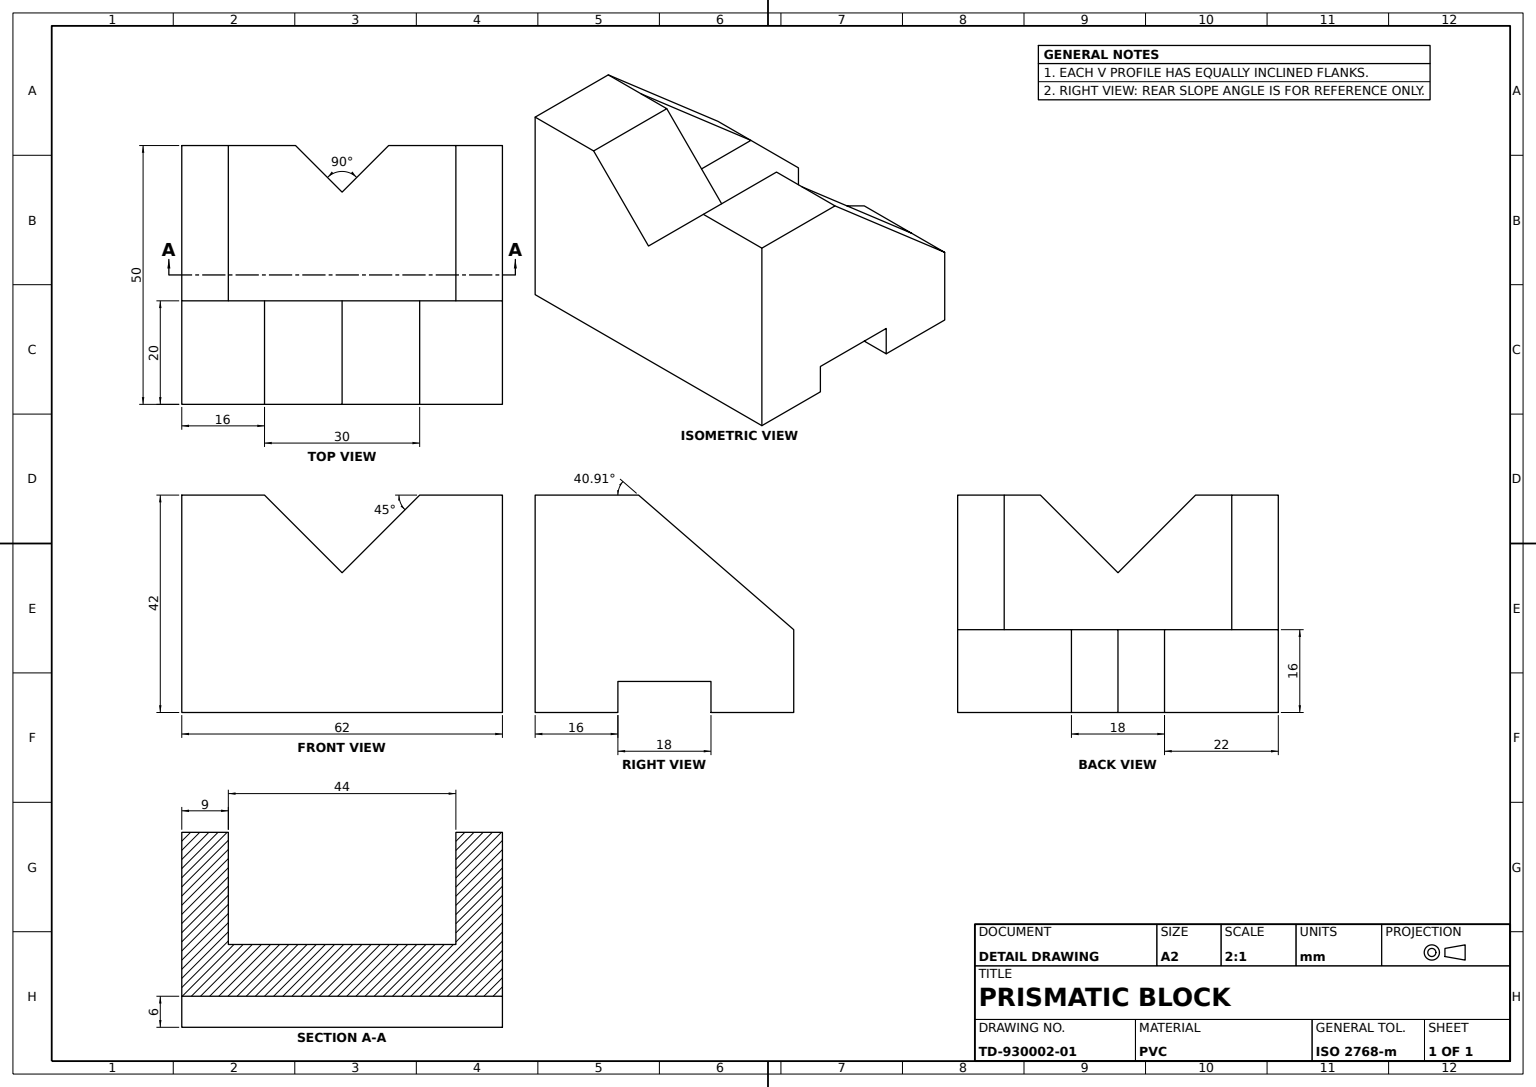
ISO-10303-21;
HEADER;
FILE_DESCRIPTION((''),'2;1');
FILE_NAME('','',(''),(''),'','','');
FILE_SCHEMA(('AUTOMOTIVE_DESIGN'));
ENDSEC;
DATA;
#1=APPLICATION_CONTEXT('');
#2=PRODUCT_CONTEXT('',#1,'mechanical');
#3=PRODUCT('','','',(#2));
#4=PRODUCT_DEFINITION_FORMATION('','',#3);
#5=PRODUCT_DEFINITION_CONTEXT('',#1,'design');
#6=PRODUCT_DEFINITION('','',#4,#5);
#7=PRODUCT_DEFINITION_SHAPE('','',#6);
#8=(LENGTH_UNIT()NAMED_UNIT(*)SI_UNIT(.MILLI.,.METRE.));
#9=(NAMED_UNIT(*)PLANE_ANGLE_UNIT()SI_UNIT($,.RADIAN.));
#10=(NAMED_UNIT(*)SI_UNIT($,.STERADIAN.)SOLID_ANGLE_UNIT());
#11=UNCERTAINTY_MEASURE_WITH_UNIT(LENGTH_MEASURE(0.005),#8,'distance_accuracy_value','');
#12=(GEOMETRIC_REPRESENTATION_CONTEXT(3)GLOBAL_UNCERTAINTY_ASSIGNED_CONTEXT((#11))GLOBAL_UNIT_ASSIGNED_CONTEXT((#8,#9,#10))REPRESENTATION_CONTEXT('',''));
#13=CARTESIAN_POINT('',(9.,25.,-21.));
#14=VERTEX_POINT('',#13);
#15=CARTESIAN_POINT('',(31.,25.,-21.));
#16=VERTEX_POINT('',#15);
#17=CARTESIAN_POINT('',(0.,25.,-21.));
#18=DIRECTION('',(1.,0.,0.));
#19=VECTOR('',#18,1000.);
#20=LINE('',#17,#19);
#21=EDGE_CURVE('',#14,#16,#20,.T.);
#22=ORIENTED_EDGE('',*,*,#21,.T.);
#23=CARTESIAN_POINT('',(31.,9.,-21.));
#24=VERTEX_POINT('',#23);
#25=CARTESIAN_POINT('',(31.,0.,-21.));
#26=DIRECTION('',(0.,1.,0.));
#27=VECTOR('',#26,1000.);
#28=LINE('',#25,#27);
#29=EDGE_CURVE('',#24,#16,#28,.T.);
#30=ORIENTED_EDGE('',*,*,#29,.F.);
#31=CARTESIAN_POINT('',(-31.,9.,-21.));
#32=VERTEX_POINT('',#31);
#33=CARTESIAN_POINT('',(0.,9.,-21.));
#34=DIRECTION('',(-1.,0.,0.));
#35=VECTOR('',#34,1000.);
#36=LINE('',#33,#35);
#37=EDGE_CURVE('',#24,#32,#36,.T.);
#38=ORIENTED_EDGE('',*,*,#37,.T.);
#39=CARTESIAN_POINT('',(-31.,25.,-21.));
#40=VERTEX_POINT('',#39);
#41=CARTESIAN_POINT('',(-31.,0.,-21.));
#42=LINE('',#41,#27);
#43=EDGE_CURVE('',#32,#40,#42,.T.);
#44=ORIENTED_EDGE('',*,*,#43,.T.);
#45=CARTESIAN_POINT('',(-9.,25.,-21.));
#46=VERTEX_POINT('',#45);
#47=EDGE_CURVE('',#40,#46,#20,.T.);
#48=ORIENTED_EDGE('',*,*,#47,.T.);
#49=CARTESIAN_POINT('',(0.,16.,-21.));
#50=VERTEX_POINT('',#49);
#51=DIRECTION('',(0.707106781,-0.707106781,0.));
#52=VECTOR('',#51,1000.);
#53=LINE('',#49,#52);
#54=EDGE_CURVE('',#46,#50,#53,.T.);
#55=ORIENTED_EDGE('',*,*,#54,.T.);
#56=CARTESIAN_POINT('',(-20.5,-4.5,-21.));
#57=DIRECTION('',(-0.707106781,-0.707106781,0.));
#58=VECTOR('',#57,1000.);
#59=LINE('',#56,#58);
#60=EDGE_CURVE('',#14,#50,#59,.T.);
#61=ORIENTED_EDGE('',*,*,#60,.F.);
#62=EDGE_LOOP('',(#22,#30,#38,#44,#48,#55,#61));
#63=FACE_BOUND('',#62,.T.);
#64=CARTESIAN_POINT('',(0.,-25.,-21.));
#65=DIRECTION('',(0.,0.,-1.));
#66=AXIS2_PLACEMENT_3D('',#64,#65,#26);
#67=PLANE('',#66);
#68=ADVANCED_FACE('',(#63),#67,.T.);
#69=CARTESIAN_POINT('',(-9.,25.,-5.));
#70=VERTEX_POINT('',#69);
#71=CARTESIAN_POINT('',(-22.,25.,-5.));
#72=VERTEX_POINT('',#71);
#73=CARTESIAN_POINT('',(0.,25.,-5.));
#74=LINE('',#73,#35);
#75=EDGE_CURVE('',#70,#72,#74,.T.);
#76=ORIENTED_EDGE('',*,*,#75,.T.);
#77=CARTESIAN_POINT('',(-22.,-5.,-5.));
#78=VERTEX_POINT('',#77);
#79=LINE('',#77,#27);
#80=EDGE_CURVE('',#78,#72,#79,.T.);
#81=ORIENTED_EDGE('',*,*,#80,.F.);
#82=CARTESIAN_POINT('',(22.,-5.,-5.));
#83=VERTEX_POINT('',#82);
#84=CARTESIAN_POINT('',(0.,-5.,-5.));
#85=LINE('',#84,#35);
#86=EDGE_CURVE('',#83,#78,#85,.T.);
#87=ORIENTED_EDGE('',*,*,#86,.F.);
#88=CARTESIAN_POINT('',(22.,25.,-5.));
#89=VERTEX_POINT('',#88);
#90=LINE('',#82,#27);
#91=EDGE_CURVE('',#83,#89,#90,.T.);
#92=ORIENTED_EDGE('',*,*,#91,.T.);
#93=CARTESIAN_POINT('',(9.,25.,-5.));
#94=VERTEX_POINT('',#93);
#95=EDGE_CURVE('',#89,#94,#74,.T.);
#96=ORIENTED_EDGE('',*,*,#95,.T.);
#97=CARTESIAN_POINT('',(0.,16.,-5.));
#98=VERTEX_POINT('',#97);
#99=LINE('',#93,#58);
#100=EDGE_CURVE('',#94,#98,#99,.T.);
#101=ORIENTED_EDGE('',*,*,#100,.T.);
#102=DIRECTION('',(-0.707106781,0.707106781,0.));
#103=VECTOR('',#102,1000.);
#104=LINE('',#97,#103);
#105=EDGE_CURVE('',#98,#70,#104,.T.);
#106=ORIENTED_EDGE('',*,*,#105,.T.);
#107=EDGE_LOOP('',(#76,#81,#87,#92,#96,#101,#106));
#108=FACE_BOUND('',#107,.T.);
#109=DIRECTION('',(0.,0.,1.));
#110=AXIS2_PLACEMENT_3D('',#84,#109,#26);
#111=PLANE('',#110);
#112=ADVANCED_FACE('',(#108),#111,.T.);
#113=CARTESIAN_POINT('',(-15.,-5.,21.));
#114=VERTEX_POINT('',#113);
#115=CARTESIAN_POINT('',(-15.,-25.,21.));
#116=VERTEX_POINT('',#115);
#117=DIRECTION('',(0.,-1.,0.));
#118=VECTOR('',#117,1000.);
#119=LINE('',#113,#118);
#120=EDGE_CURVE('',#114,#116,#119,.T.);
#121=ORIENTED_EDGE('',*,*,#120,.T.);
#122=CARTESIAN_POINT('',(0.,-25.,6.));
#123=VERTEX_POINT('',#122);
#124=DIRECTION('',(0.707106781,0.,-0.707106781));
#125=VECTOR('',#124,1000.);
#126=LINE('',#122,#125);
#127=EDGE_CURVE('',#116,#123,#126,.T.);
#128=ORIENTED_EDGE('',*,*,#127,.T.);
#129=CARTESIAN_POINT('',(0.,-5.,6.));
#130=VERTEX_POINT('',#129);
#131=LINE('',#129,#118);
#132=EDGE_CURVE('',#130,#123,#131,.T.);
#133=ORIENTED_EDGE('',*,*,#132,.F.);
#134=DIRECTION('',(-0.707106781,0.,0.707106781));
#135=VECTOR('',#134,1000.);
#136=LINE('',#129,#135);
#137=EDGE_CURVE('',#130,#114,#136,.T.);
#138=ORIENTED_EDGE('',*,*,#137,.T.);
#139=EDGE_LOOP('',(#121,#128,#133,#138));
#140=FACE_BOUND('',#139,.T.);
#141=DIRECTION('',(0.707106781,0.,0.707106781));
#142=AXIS2_PLACEMENT_3D('',#129,#141,#134);
#143=PLANE('',#142);
#144=ADVANCED_FACE('',(#140),#143,.T.);
#145=CARTESIAN_POINT('',(15.,-25.,21.));
#146=VERTEX_POINT('',#145);
#147=CARTESIAN_POINT('',(7.5,-25.,13.5));
#148=DIRECTION('',(-0.707106781,0.,-0.707106781));
#149=VECTOR('',#148,1000.);
#150=LINE('',#147,#149);
#151=EDGE_CURVE('',#146,#123,#150,.T.);
#152=ORIENTED_EDGE('',*,*,#151,.T.);
#153=ORIENTED_EDGE('',*,*,#127,.F.);
#154=CARTESIAN_POINT('',(-31.,-25.,21.));
#155=VERTEX_POINT('',#154);
#156=CARTESIAN_POINT('',(0.,-25.,21.));
#157=LINE('',#156,#19);
#158=EDGE_CURVE('',#155,#116,#157,.T.);
#159=ORIENTED_EDGE('',*,*,#158,.F.);
#160=CARTESIAN_POINT('',(-31.,-25.,-21.));
#161=VERTEX_POINT('',#160);
#162=CARTESIAN_POINT('',(-31.,-25.,0.));
#163=VECTOR('',#65,1000.);
#164=LINE('',#162,#163);
#165=EDGE_CURVE('',#155,#161,#164,.T.);
#166=ORIENTED_EDGE('',*,*,#165,.T.);
#167=CARTESIAN_POINT('',(31.,-25.,-21.));
#168=VERTEX_POINT('',#167);
#169=LINE('',#64,#19);
#170=EDGE_CURVE('',#161,#168,#169,.T.);
#171=ORIENTED_EDGE('',*,*,#170,.T.);
#172=CARTESIAN_POINT('',(31.,-25.,21.));
#173=VERTEX_POINT('',#172);
#174=CARTESIAN_POINT('',(31.,-25.,0.));
#175=LINE('',#174,#163);
#176=EDGE_CURVE('',#173,#168,#175,.T.);
#177=ORIENTED_EDGE('',*,*,#176,.F.);
#178=EDGE_CURVE('',#146,#173,#157,.T.);
#179=ORIENTED_EDGE('',*,*,#178,.F.);
#180=EDGE_LOOP('',(#152,#153,#159,#166,#171,#177,#179));
#181=FACE_BOUND('',#180,.T.);
#182=AXIS2_PLACEMENT_3D('',#156,#117,#65);
#183=PLANE('',#182);
#184=ADVANCED_FACE('',(#181),#183,.T.);
#185=CARTESIAN_POINT('',(15.,-5.,21.));
#186=VERTEX_POINT('',#185);
#187=LINE('',#185,#149);
#188=EDGE_CURVE('',#186,#130,#187,.T.);
#189=ORIENTED_EDGE('',*,*,#188,.T.);
#190=ORIENTED_EDGE('',*,*,#132,.T.);
#191=ORIENTED_EDGE('',*,*,#151,.F.);
#192=LINE('',#185,#118);
#193=EDGE_CURVE('',#186,#146,#192,.T.);
#194=ORIENTED_EDGE('',*,*,#193,.F.);
#195=EDGE_LOOP('',(#189,#190,#191,#194));
#196=FACE_BOUND('',#195,.T.);
#197=AXIS2_PLACEMENT_3D('',#185,#134,#148);
#198=PLANE('',#197);
#199=ADVANCED_FACE('',(#196),#198,.T.);
#200=CARTESIAN_POINT('',(-31.,-5.,21.));
#201=VERTEX_POINT('',#200);
#202=CARTESIAN_POINT('',(-31.,0.,21.));
#203=LINE('',#202,#118);
#204=EDGE_CURVE('',#201,#155,#203,.T.);
#205=ORIENTED_EDGE('',*,*,#204,.F.);
#206=CARTESIAN_POINT('',(-31.,25.,-5.));
#207=VERTEX_POINT('',#206);
#208=CARTESIAN_POINT('',(-31.,8.248731,9.517766));
#209=DIRECTION('',(0.,-0.755689083,0.654930538));
#210=VECTOR('',#209,1000.);
#211=LINE('',#208,#210);
#212=EDGE_CURVE('',#207,#201,#211,.T.);
#213=ORIENTED_EDGE('',*,*,#212,.F.);
#214=CARTESIAN_POINT('',(-31.,25.,0.));
#215=VECTOR('',#109,1000.);
#216=LINE('',#214,#215);
#217=EDGE_CURVE('',#40,#207,#216,.T.);
#218=ORIENTED_EDGE('',*,*,#217,.F.);
#219=ORIENTED_EDGE('',*,*,#43,.F.);
#220=CARTESIAN_POINT('',(-31.,9.,-15.));
#221=VERTEX_POINT('',#220);
#222=LINE('',#31,#215);
#223=EDGE_CURVE('',#32,#221,#222,.T.);
#224=ORIENTED_EDGE('',*,*,#223,.T.);
#225=CARTESIAN_POINT('',(-31.,-9.,-15.));
#226=VERTEX_POINT('',#225);
#227=LINE('',#225,#27);
#228=EDGE_CURVE('',#226,#221,#227,.T.);
#229=ORIENTED_EDGE('',*,*,#228,.F.);
#230=CARTESIAN_POINT('',(-31.,-9.,-21.));
#231=VERTEX_POINT('',#230);
#232=CARTESIAN_POINT('',(-31.,-9.,0.));
#233=LINE('',#232,#215);
#234=EDGE_CURVE('',#231,#226,#233,.T.);
#235=ORIENTED_EDGE('',*,*,#234,.F.);
#236=EDGE_CURVE('',#161,#231,#42,.T.);
#237=ORIENTED_EDGE('',*,*,#236,.F.);
#238=ORIENTED_EDGE('',*,*,#165,.F.);
#239=EDGE_LOOP('',(#205,#213,#218,#219,#224,#229,#235,#237,#238));
#240=FACE_BOUND('',#239,.T.);
#241=CARTESIAN_POINT('',(-31.,0.,0.));
#242=AXIS2_PLACEMENT_3D('',#241,#18,#26);
#243=PLANE('',#242);
#244=ADVANCED_FACE('',(#240),#243,.F.);
#245=CARTESIAN_POINT('',(31.,25.,-5.));
#246=VERTEX_POINT('',#245);
#247=LINE('',#73,#19);
#248=EDGE_CURVE('',#89,#246,#247,.T.);
#249=ORIENTED_EDGE('',*,*,#248,.F.);
#250=CARTESIAN_POINT('',(22.,-5.,21.));
#251=VERTEX_POINT('',#250);
#252=CARTESIAN_POINT('',(22.,8.248731,9.517766));
#253=LINE('',#252,#210);
#254=EDGE_CURVE('',#89,#251,#253,.T.);
#255=ORIENTED_EDGE('',*,*,#254,.T.);
#256=CARTESIAN_POINT('',(31.,-5.,21.));
#257=VERTEX_POINT('',#256);
#258=CARTESIAN_POINT('',(0.,-5.,21.));
#259=LINE('',#258,#19);
#260=EDGE_CURVE('',#251,#257,#259,.T.);
#261=ORIENTED_EDGE('',*,*,#260,.T.);
#262=CARTESIAN_POINT('',(31.,8.248731,9.517766));
#263=LINE('',#262,#210);
#264=EDGE_CURVE('',#246,#257,#263,.T.);
#265=ORIENTED_EDGE('',*,*,#264,.F.);
#266=EDGE_LOOP('',(#249,#255,#261,#265));
#267=FACE_BOUND('',#266,.T.);
#268=DIRECTION('',(0.,0.654930538,0.755689083));
#269=AXIS2_PLACEMENT_3D('',#73,#268,#209);
#270=PLANE('',#269);
#271=ADVANCED_FACE('',(#267),#270,.T.);
#272=ORIENTED_EDGE('',*,*,#37,.F.);
#273=CARTESIAN_POINT('',(31.,9.,-15.));
#274=VERTEX_POINT('',#273);
#275=LINE('',#23,#215);
#276=EDGE_CURVE('',#24,#274,#275,.T.);
#277=ORIENTED_EDGE('',*,*,#276,.T.);
#278=LINE('',#273,#35);
#279=EDGE_CURVE('',#274,#221,#278,.T.);
#280=ORIENTED_EDGE('',*,*,#279,.T.);
#281=ORIENTED_EDGE('',*,*,#223,.F.);
#282=EDGE_LOOP('',(#272,#277,#280,#281));
#283=FACE_BOUND('',#282,.T.);
#284=AXIS2_PLACEMENT_3D('',#23,#117,#109);
#285=PLANE('',#284);
#286=ADVANCED_FACE('',(#283),#285,.T.);
#287=ORIENTED_EDGE('',*,*,#178,.T.);
#288=CARTESIAN_POINT('',(31.,0.,21.));
#289=LINE('',#288,#118);
#290=EDGE_CURVE('',#257,#173,#289,.T.);
#291=ORIENTED_EDGE('',*,*,#290,.F.);
#292=ORIENTED_EDGE('',*,*,#260,.F.);
#293=LINE('',#258,#35);
#294=EDGE_CURVE('',#251,#186,#293,.T.);
#295=ORIENTED_EDGE('',*,*,#294,.T.);
#296=ORIENTED_EDGE('',*,*,#193,.T.);
#297=EDGE_LOOP('',(#287,#291,#292,#295,#296));
#298=FACE_BOUND('',#297,.T.);
#299=AXIS2_PLACEMENT_3D('',#258,#109,#117);
#300=PLANE('',#299);
#301=ADVANCED_FACE('',(#298),#300,.T.);
#302=ORIENTED_EDGE('',*,*,#91,.F.);
#303=LINE('',#250,#163);
#304=EDGE_CURVE('',#251,#83,#303,.T.);
#305=ORIENTED_EDGE('',*,*,#304,.F.);
#306=ORIENTED_EDGE('',*,*,#254,.F.);
#307=EDGE_LOOP('',(#302,#305,#306));
#308=FACE_BOUND('',#307,.T.);
#309=CARTESIAN_POINT('',(22.,0.,0.));
#310=AXIS2_PLACEMENT_3D('',#309,#18,#26);
#311=PLANE('',#310);
#312=ADVANCED_FACE('',(#308),#311,.F.);
#313=CARTESIAN_POINT('',(31.,25.,0.));
#314=LINE('',#313,#215);
#315=EDGE_CURVE('',#16,#246,#314,.T.);
#316=ORIENTED_EDGE('',*,*,#315,.F.);
#317=ORIENTED_EDGE('',*,*,#21,.F.);
#318=LINE('',#13,#163);
#319=EDGE_CURVE('',#94,#14,#318,.T.);
#320=ORIENTED_EDGE('',*,*,#319,.F.);
#321=ORIENTED_EDGE('',*,*,#95,.F.);
#322=ORIENTED_EDGE('',*,*,#248,.T.);
#323=EDGE_LOOP('',(#316,#317,#320,#321,#322));
#324=FACE_BOUND('',#323,.T.);
#325=AXIS2_PLACEMENT_3D('',#17,#26,#109);
#326=PLANE('',#325);
#327=ADVANCED_FACE('',(#324),#326,.T.);
#328=ORIENTED_EDGE('',*,*,#212,.T.);
#329=CARTESIAN_POINT('',(-22.,-5.,21.));
#330=VERTEX_POINT('',#329);
#331=EDGE_CURVE('',#201,#330,#259,.T.);
#332=ORIENTED_EDGE('',*,*,#331,.T.);
#333=CARTESIAN_POINT('',(-22.,8.248731,9.517766));
#334=LINE('',#333,#210);
#335=EDGE_CURVE('',#72,#330,#334,.T.);
#336=ORIENTED_EDGE('',*,*,#335,.F.);
#337=EDGE_CURVE('',#207,#72,#247,.T.);
#338=ORIENTED_EDGE('',*,*,#337,.F.);
#339=EDGE_LOOP('',(#328,#332,#336,#338));
#340=FACE_BOUND('',#339,.T.);
#341=ADVANCED_FACE('',(#340),#270,.T.);
#342=CARTESIAN_POINT('',(31.,-9.,-15.));
#343=VERTEX_POINT('',#342);
#344=LINE('',#342,#35);
#345=EDGE_CURVE('',#343,#226,#344,.T.);
#346=ORIENTED_EDGE('',*,*,#345,.T.);
#347=ORIENTED_EDGE('',*,*,#228,.T.);
#348=ORIENTED_EDGE('',*,*,#279,.F.);
#349=LINE('',#342,#27);
#350=EDGE_CURVE('',#343,#274,#349,.T.);
#351=ORIENTED_EDGE('',*,*,#350,.F.);
#352=EDGE_LOOP('',(#346,#347,#348,#351));
#353=FACE_BOUND('',#352,.T.);
#354=AXIS2_PLACEMENT_3D('',#342,#109,#26);
#355=PLANE('',#354);
#356=ADVANCED_FACE('',(#353),#355,.F.);
#357=ORIENTED_EDGE('',*,*,#345,.F.);
#358=CARTESIAN_POINT('',(31.,-9.,-21.));
#359=VERTEX_POINT('',#358);
#360=LINE('',#342,#163);
#361=EDGE_CURVE('',#343,#359,#360,.T.);
#362=ORIENTED_EDGE('',*,*,#361,.T.);
#363=LINE('',#358,#35);
#364=EDGE_CURVE('',#359,#231,#363,.T.);
#365=ORIENTED_EDGE('',*,*,#364,.T.);
#366=ORIENTED_EDGE('',*,*,#234,.T.);
#367=EDGE_LOOP('',(#357,#362,#365,#366));
#368=FACE_BOUND('',#367,.T.);
#369=AXIS2_PLACEMENT_3D('',#342,#26,#65);
#370=PLANE('',#369);
#371=ADVANCED_FACE('',(#368),#370,.T.);
#372=LINE('',#69,#163);
#373=EDGE_CURVE('',#70,#46,#372,.T.);
#374=ORIENTED_EDGE('',*,*,#373,.T.);
#375=ORIENTED_EDGE('',*,*,#47,.F.);
#376=ORIENTED_EDGE('',*,*,#217,.T.);
#377=ORIENTED_EDGE('',*,*,#337,.T.);
#378=ORIENTED_EDGE('',*,*,#75,.F.);
#379=EDGE_LOOP('',(#374,#375,#376,#377,#378));
#380=FACE_BOUND('',#379,.T.);
#381=ADVANCED_FACE('',(#380),#326,.T.);
#382=ORIENTED_EDGE('',*,*,#335,.T.);
#383=LINE('',#329,#163);
#384=EDGE_CURVE('',#330,#78,#383,.T.);
#385=ORIENTED_EDGE('',*,*,#384,.T.);
#386=ORIENTED_EDGE('',*,*,#80,.T.);
#387=EDGE_LOOP('',(#382,#385,#386));
#388=FACE_BOUND('',#387,.T.);
#389=CARTESIAN_POINT('',(-22.,0.,0.));
#390=AXIS2_PLACEMENT_3D('',#389,#18,#26);
#391=PLANE('',#390);
#392=ADVANCED_FACE('',(#388),#391,.T.);
#393=ORIENTED_EDGE('',*,*,#29,.T.);
#394=ORIENTED_EDGE('',*,*,#315,.T.);
#395=ORIENTED_EDGE('',*,*,#264,.T.);
#396=ORIENTED_EDGE('',*,*,#290,.T.);
#397=ORIENTED_EDGE('',*,*,#176,.T.);
#398=EDGE_CURVE('',#168,#359,#28,.T.);
#399=ORIENTED_EDGE('',*,*,#398,.T.);
#400=ORIENTED_EDGE('',*,*,#361,.F.);
#401=ORIENTED_EDGE('',*,*,#350,.T.);
#402=ORIENTED_EDGE('',*,*,#276,.F.);
#403=EDGE_LOOP('',(#393,#394,#395,#396,#397,#399,#400,#401,#402));
#404=FACE_BOUND('',#403,.T.);
#405=CARTESIAN_POINT('',(31.,0.,0.));
#406=AXIS2_PLACEMENT_3D('',#405,#18,#26);
#407=PLANE('',#406);
#408=ADVANCED_FACE('',(#404),#407,.T.);
#409=ORIENTED_EDGE('',*,*,#137,.F.);
#410=ORIENTED_EDGE('',*,*,#188,.F.);
#411=ORIENTED_EDGE('',*,*,#294,.F.);
#412=ORIENTED_EDGE('',*,*,#304,.T.);
#413=ORIENTED_EDGE('',*,*,#86,.T.);
#414=ORIENTED_EDGE('',*,*,#384,.F.);
#415=EDGE_CURVE('',#114,#330,#293,.T.);
#416=ORIENTED_EDGE('',*,*,#415,.F.);
#417=EDGE_LOOP('',(#409,#410,#411,#412,#413,#414,#416));
#418=FACE_BOUND('',#417,.T.);
#419=AXIS2_PLACEMENT_3D('',#258,#26,#65);
#420=PLANE('',#419);
#421=ADVANCED_FACE('',(#418),#420,.T.);
#422=ORIENTED_EDGE('',*,*,#398,.F.);
#423=ORIENTED_EDGE('',*,*,#170,.F.);
#424=ORIENTED_EDGE('',*,*,#236,.T.);
#425=ORIENTED_EDGE('',*,*,#364,.F.);
#426=EDGE_LOOP('',(#422,#423,#424,#425));
#427=FACE_BOUND('',#426,.T.);
#428=ADVANCED_FACE('',(#427),#67,.T.);
#429=ORIENTED_EDGE('',*,*,#331,.F.);
#430=ORIENTED_EDGE('',*,*,#204,.T.);
#431=ORIENTED_EDGE('',*,*,#158,.T.);
#432=ORIENTED_EDGE('',*,*,#120,.F.);
#433=ORIENTED_EDGE('',*,*,#415,.T.);
#434=EDGE_LOOP('',(#429,#430,#431,#432,#433));
#435=FACE_BOUND('',#434,.T.);
#436=ADVANCED_FACE('',(#435),#300,.T.);
#437=ORIENTED_EDGE('',*,*,#100,.F.);
#438=ORIENTED_EDGE('',*,*,#319,.T.);
#439=ORIENTED_EDGE('',*,*,#60,.T.);
#440=LINE('',#97,#163);
#441=EDGE_CURVE('',#98,#50,#440,.T.);
#442=ORIENTED_EDGE('',*,*,#441,.F.);
#443=EDGE_LOOP('',(#437,#438,#439,#442));
#444=FACE_BOUND('',#443,.T.);
#445=AXIS2_PLACEMENT_3D('',#93,#51,#57);
#446=PLANE('',#445);
#447=ADVANCED_FACE('',(#444),#446,.F.);
#448=ORIENTED_EDGE('',*,*,#54,.F.);
#449=ORIENTED_EDGE('',*,*,#373,.F.);
#450=ORIENTED_EDGE('',*,*,#105,.F.);
#451=ORIENTED_EDGE('',*,*,#441,.T.);
#452=EDGE_LOOP('',(#448,#449,#450,#451));
#453=FACE_BOUND('',#452,.T.);
#454=AXIS2_PLACEMENT_3D('',#97,#57,#102);
#455=PLANE('',#454);
#456=ADVANCED_FACE('',(#453),#455,.F.);
#457=CLOSED_SHELL('',(#68,#112,#144,#184,#199,#244,#271,#286,#301,#312,#327,#341,#356,#371,#381,#392,#408,#421,#428,#436,#447,#456));
#458=MANIFOLD_SOLID_BREP('',#457);
#459=ADVANCED_BREP_SHAPE_REPRESENTATION('',(#458),#12);
#460=SHAPE_DEFINITION_REPRESENTATION(#7,#459);
ENDSEC;
END-ISO-10303-21;
